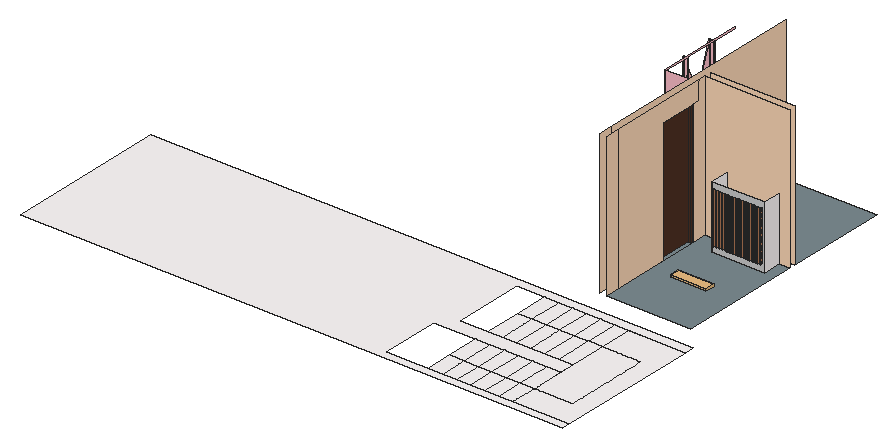
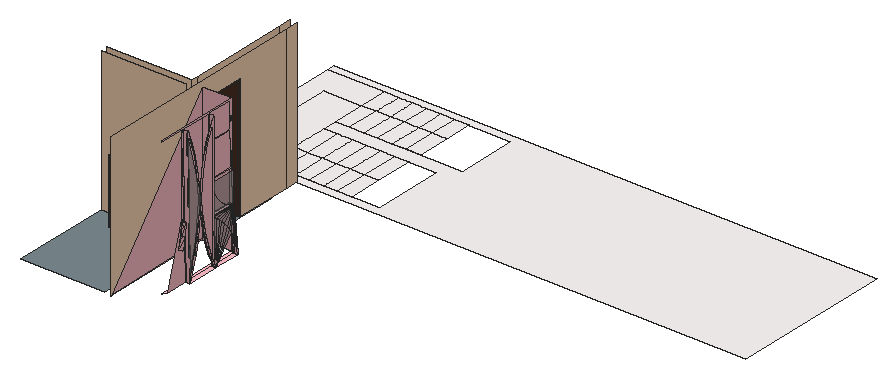
# SketchUp Ruby script. Lengths in inches.
U = 1.inch
M = Sketchup.active_model
def pt(a) = Geom::Point3d.new(a.map { |v| v * U })
def face(e, loops, mat)
  f = e.add_face(loops[0].map { |a| pt(a) })
  loops[1..].each { |l| e.add_face(l.map { |a| pt(a) }).erase! }
  f.material = f.back_material = mat if mat
  f
end
# faces: each face lists its corners as indices into pts; further lists are holes
def faces(e, pts, list, mat = nil) = list.each { |f| face(e, (f[0].is_a?(Array) ? f : [f]).map { |l| l.map { |i| pts[i] } }, mat) }
# xy, xz, yz: faces in a plane at the given z, y or x. An outline is a flat list of corners, or four numbers for a rectangle; further outlines are holes
def ring(l) = l.size == 4 ? [[l[0], l[1]], [l[2], l[1]], [l[2], l[3]], [l[0], l[3]]] : l.each_slice(2).to_a
def flat(e, list, mat, &to3) = list.each { |f| face(e, (f[0].is_a?(Array) ? f : [f]).map { |l| ring(l).map { |u, v| to3.(u, v) } }, mat) }
def xy(e, z, list, mat = nil) = flat(e, list, mat) { |x, y| [x, y, z] }
def xz(e, y, list, mat = nil) = flat(e, list, mat) { |x, z| [x, y, z] }
def yz(e, x, list, mat = nil) = flat(e, list, mat) { |y, z| [x, y, z] }
def lines(e, pts, list) = list.each { |a, b| e.add_line(pt(pts[a]), pt(pts[b])) }
# prism: a flat outline (further loops are holes) pulled along v
def prism(e, loops, v, mat = nil)
  f = face(e, loops, mat); d = Geom::Vector3d.new(v.map { |x| x * U })
  f.pushpull(f.normal.samedirection?(d) ? d.length : -d.length)
end
def box(e, o, s, mat = nil) = prism(e, [[o, [o[0] + s[0], o[1], o[2]], [o[0] + s[0], o[1] + s[1], o[2]], [o[0], o[1] + s[1], o[2]]]], [0, 0, s[2]], mat)
def at(x, y, z, deg = 0) = Geom::Transformation.translation(pt([x, y, z])) * Geom::Transformation.rotation(ORIGIN, Z_AXIS, deg.degrees)
def axes(o, x, y, z) = Geom::Transformation.new([*x, 0, *y, 0, *z, 0, *pt(o).to_a, 1])
def part(name) = M.definitions.add(name)
# library, detail: a bought-in or finely detailed component or shape, given as its bounding box
def library(name, o, s) = part(name).tap { |d| box(d.entities, o, s) }
def detail(e, o, s) = box(e.add_group.entities, o, s)
def put(e, d, t, mat = nil) = e.add_instance(d, t).tap { |i| i.material = mat if mat }
def group(e, t, mat = nil) = e.add_group.tap { |g| g.transformation = t; g.material = mat if mat }.entities
root = M.entities
M.materials.add("Polis06_194").color = [79, 50, 36]
M.materials.add("[0006_Pink]").color = [255, 192, 203]
M.materials.add("[0007_MistyRose]").color = [255, 228, 225]
M.materials.add("[0010_Snow]").color = [255, 250, 250]
M.materials.add("[0027_PeachPuff]").color = [255, 218, 185]
M.materials.add("[Carrera Marble]").color = [207, 207, 207]
M.materials.add("[Concrete Pavers Block Multi]").color = [124, 140, 145]
M.materials.add("[Translucent Glass Gray]").color = [128, 128, 128]
M.materials["[Translucent Glass Gray]"].alpha = 0.5
M.materials.add("[Wood Veneer 02]").color = [190, 128, 91]
c1 = part("Interior door")
xy(c1.entities,0,[[0,0,4.72,1.18],[0,34.25,4.72,35.43]],"Polis06_194")
xy(c1.entities,85.26,[[0,1.18,4.72,34.25]],"Polis06_194")
xy(c1.entities,86.61,[[0,0,4.72,35.43]],"Polis06_194")
xz(c1.entities,0,[[0,0,4.72,86.61]],"Polis06_194")
xz(c1.entities,1.18,[[0,0,2.36,85.26],[2.36,0,4.72,85.26]],"Polis06_194")
xz(c1.entities,34.25,[[0,0,4.72,85.26]],"Polis06_194")
xz(c1.entities,35.43,[[0,0,4.72,86.61]],"Polis06_194")
yz(c1.entities,0,[[0,0,1.18,86.61],[34.25,0,35.43,86.61],[1.18,85.26,34.25,86.61]],"Polis06_194")
yz(c1.entities,2.36,[[1.18,0,34.25,0,34.25,85.21,1.18,85.26]],"Polis06_194")
yz(c1.entities,4.72,[[0,0,1.18,86.61],[34.25,0,35.43,86.61],[1.18,85.26,34.25,86.61]],"Polis06_194")
c2 = library("toilet 2",[0.13,0,0],[30.44,8.22,2])
xy(root,-7.5625,[[109.5625,0,571.5625,0,571.5625,6.25,415.5625,6.25,415.5625,57.9375,523.5625,57.9375,523.5625,70.375,427.5625,70.375,427.5625,130.875,571.5625,130.875,571.5625,138.9375,109.5625,138.9375],[451.5625,6.25,463.5625,29.875],[463.5625,6.25,475.5625,29.875],[475.5625,6.25,487.5625,29.875],[487.5625,6.25,499.5625,29.875],
  [499.5625,6.25,511.5625,29.875],[511.5625,6.25,523.5625,29.875],[523.5625,6.25,571.5625,6.25,571.5625,130.875,523.5625,130.875,523.5625,102.3125,556.33,102.3125,556.33,29.875,523.5625,29.875],[451.5625,29.875,463.5625,57.9375],[463.5625,29.875,475.5625,57.9375],
  [475.5625,29.875,487.5625,57.9375],[487.5625,29.875,499.5625,57.9375],[499.5625,29.875,511.5625,57.9375],[511.5625,29.875,523.5625,57.9375],[523.5625,29.875,556.33,102.3125],
  [451.5625,70.375,463.5625,102.3125],[463.5625,70.375,475.5625,102.3125],[475.5625,70.375,487.5625,102.3125],[487.5625,70.375,499.5625,102.3125],[499.5625,70.375,511.5625,102.3125],
  [511.5625,70.375,523.5625,102.3125],[451.5625,102.3125,463.5625,130.875],[463.5625,102.3125,475.5625,130.875],[475.5625,102.3125,487.5625,130.875],[487.5625,102.3125,499.5625,130.875],
  [499.5625,102.3125,511.5625,130.875],[511.5625,102.3125,523.5625,130.875]],"[0010_Snow]")
xy(root,0,[[508.61,237.66,553.2,252.9375],[500.21,258.9375,543.78,274.78]],"[0010_Snow]")
xy(root,0,[[484.5625,240.51,490.5625,246.2]],"[0027_PeachPuff]")
xy(root,0,[[490.5625,147.9375,562.5625,147.9375,562.5625,252.9375,553.2,252.9375,553.2,237.66,508.61,237.66,508.61,252.9375,490.5625,252.9375],[483.52,177.19,490.5625,240.51],[490.5625,258.9375,500.21,258.9375,500.21,274.78,543.78,274.78,543.78,258.9375,562.5625,258.9375,562.5625,345.21,490.5625,345.21]],"[Concrete Pavers Block Multi]")
xy(root,0.5,[[453.17,250.71,456.54,272.96],[453.17,273.46,456.54,301.21]],"[0006_Pink]")
xy(root,5.99,[[510.4375,236.375,511.58,237.09],[512.87,236.375,514.01,237.09],[515.3,236.375,516.4375,237.09],[517.73,236.375,518.87,237.09],[520.16,236.375,521.3,237.09],
  [522.59,236.375,523.73,237.09],[525.02,236.375,526.16,237.09],[527.45,236.375,528.59,237.09],[529.88,236.375,531.02,237.09],[531.83,236.375,532.97,237.09],
  [534.125,236.375,535.26,237.09],[536.42,236.375,537.55,237.09],[538.71,236.375,539.85,237.09],[541,236.375,542.14,237.09],[543.3,236.375,544.43,237.09],
  [545.59,236.375,546.73,237.09],[547.88,236.375,549.02,237.09],[550.18,236.375,551.3125,237.09],[510.4375,237.09,531.02,237.66],[531.51,237.09,551.3125,237.66]],"[0010_Snow]")
xy(root,6.2,[[502.06,274.78,521.41,275.36],[521.88,274.78,542,275.36],[502.06,275.36,503.17,276.11],[504.3,275.36,505.41,276.11],[506.54,275.36,507.65,276.11],
  [508.78,275.36,509.89,276.11],[511.02,275.36,512.13,276.11],[513.26,275.36,514.37,276.11],[515.5,275.36,516.61,276.11],[517.74,275.36,518.85,276.11],
  [519.98,275.36,521.09,276.11],[521.88,275.36,522.99,276.11],[524.26,275.36,525.37,276.11],[526.63,275.36,527.74,276.11],[529.01,275.36,530.12,276.11],
  [531.38,275.36,532.5,276.11],[533.76,275.36,534.87,276.11],[536.13,275.36,537.25,276.11],[538.51,275.36,539.62,276.11],[540.89,275.36,542,276.11]],"[0010_Snow]")
xy(root,37.375,[[456.0625,250.71,459.4375,272.96]],"[0006_Pink]")
xy(root,37.875,[[456.0625,250.71,459.4375,272.96]],"[0006_Pink]")
xz(root,207.77,[[484.5625,0,490.5625,105.5625]],"[0027_PeachPuff]")
xz(root,236.375,[[510.4375,5.99,511.58,48.56],[512.87,5.99,514.01,48.56],[515.3,5.99,516.4375,48.56],[517.73,5.99,518.87,48.56],[520.16,5.99,521.3,48.56],
  [522.59,5.99,523.73,48.56],[525.02,5.99,526.16,48.56],[527.45,5.99,528.59,48.56],[529.88,5.99,531.02,48.56],[531.83,5.99,532.97,48.56],
  [534.125,5.99,535.26,48.56],[536.42,5.99,537.55,48.56],[538.71,5.99,539.85,48.56],[541,5.99,542.14,48.56],[543.3,5.99,544.43,48.56],
  [545.59,5.99,546.73,48.56],[547.88,5.99,549.02,48.56],[550.18,5.99,551.3125,48.56]],"[Wood Veneer 02]")
xz(root,237.09,[[510.4375,5.99,511.58,48.56],[511.58,5.99,512.87,48.56],[512.87,5.99,514.01,48.56],[514.01,5.99,515.3,48.56],[515.3,5.99,516.4375,48.56],
  [516.4375,5.99,517.73,48.56],[517.73,5.99,518.87,48.56],[518.87,5.99,520.16,48.56],[520.16,5.99,521.3,48.56],[521.3,5.99,522.59,48.56],
  [522.59,5.99,523.73,48.56],[523.73,5.99,525.02,48.56],[525.02,5.99,526.16,48.56],[526.16,5.99,527.45,48.56],[527.45,5.99,528.59,48.56],
  [529.88,5.99,531.02,48.56],[531.51,5.99,531.83,48.56],[531.83,5.99,532.97,48.56],[532.97,5.99,534.125,48.56],[534.125,5.99,535.26,48.56],
  [535.26,5.99,536.42,48.56],[536.42,5.99,537.55,48.56],[537.55,5.99,538.71,48.56],[538.71,5.99,539.85,48.56],[539.85,5.99,541,48.56],
  [541,5.99,542.14,48.56],[542.14,5.99,543.3,48.56],[543.3,5.99,544.43,48.56],[544.43,5.99,545.59,48.56],[545.59,5.99,546.73,48.56],
  [546.73,5.99,547.88,48.56],[547.88,5.99,549.02,48.56],[549.02,5.99,550.18,48.56],[550.18,5.99,551.3125,48.56]],"[0010_Snow]")
xz(root,237.09,[[528.59,5.99,529.88,48.56]],"[Wood Veneer 02]")
xz(root,237.66,[[[508.61,0,553.2,53.66],[510.4375,5.99,531.02,48.56],[531.51,5.99,551.3125,48.56]]],"[Carrera Marble]")
xz(root,240.51,[[484.5625,0,490.5625,105.5625]],"[0027_PeachPuff]")
xz(root,249.21,[[459.4375,0,484.5625,0,484.33,0.5,484.5625,116.8125,459.4375,116.8125]],"[0006_Pink]")
xz(root,250.71,[[453.17,0.5,456.54,0.5,457.47,37.375,456.0625,37.375],[456.54,0.5,459.4375,37.375,457.47,37.375],[457.47,37.375,459.4375,37.375,459.4375,37.875,457.48,37.875],[456.0625,37.875,457.48,37.875,458.13,63.875,456.0625,63.875],[457.48,37.875,459.4375,37.875,459.4375,63.875,458.13,63.875]],"[0006_Pink]")
xz(root,252.9375,[[490.5625,0,562.5625,121.1875]],"[0027_PeachPuff]")
xz(root,252.9375,[[508.61,0,553.2,53.66]],"[Wood Veneer 02]")
xz(root,258.9375,[[490.5625,0,562.5625,121.1875]],"[0027_PeachPuff]")
xz(root,258.9375,[[500.21,0,543.78,55.54]],"[Wood Veneer 02]")
xz(root,272.96,[[453.17,0.5,456.0625,37.375,459.4375,37.375,456.54,0.5],[456.0625,37.875,459.4375,63.875]],"[0006_Pink]")
xz(root,273.46,[[455.3125,0.5,456.54,0.5,459.4375,115.8125,456.0625,115.8125,456.0625,114.75,455.3125,114.75]],"[0006_Pink]")
xz(root,273.86,[[455.3125,2.32,456.0625,112.97]],"[0006_Pink]")
xz(root,274.78,[[[500.21,0,543.78,55.54],[521.88,6.2,542,50.26],[502.06,6.2,521.41,50.26]]],"[0010_Snow]")
xz(root,275.36,[[502.06,6.2,503.17,50.26],[503.17,6.2,504.3,50.26],[504.3,6.2,505.41,50.26],[505.41,6.2,506.54,50.26],[506.54,6.2,507.65,50.26],
  [507.65,6.2,508.78,50.26],[508.78,6.2,509.89,50.26],[509.89,6.2,511.02,50.26],[511.02,6.2,512.13,50.26],[512.13,6.2,513.26,50.26],
  [513.26,6.2,514.37,50.26],[514.37,6.2,515.5,50.26],[515.5,6.2,516.61,50.26],[516.61,6.2,517.74,50.26],[517.74,6.2,518.85,50.26],
  [518.85,6.2,519.98,50.26],[519.98,6.2,521.09,50.26],[521.09,6.2,521.41,50.26],[521.88,6.2,522.99,50.26],[522.99,6.2,524.26,50.26],
  [524.26,6.2,525.37,50.26],[525.37,6.2,526.63,50.26],[526.63,6.2,527.74,50.26],[527.74,6.2,529.01,50.26],[529.01,6.2,530.12,50.26],
  [530.12,6.2,531.38,50.26],[531.38,6.2,532.5,50.26],[532.5,6.2,533.76,50.26],[533.76,6.2,534.87,50.26],[534.87,6.2,536.13,50.26],
  [536.13,6.2,537.25,50.26],[537.25,6.2,538.51,50.26],[538.51,6.2,539.62,50.26],[539.62,6.2,540.89,50.26]],"[0010_Snow]")
xz(root,275.36,[[540.89,6.2,542,50.26]],"[Wood Veneer 02]")
xz(root,276.11,[[502.06,6.2,503.17,50.26],[504.3,6.2,505.41,50.26],[506.54,6.2,507.65,50.26],[508.78,6.2,509.89,50.26],[511.02,6.2,512.13,50.26],
  [513.26,6.2,514.37,50.26],[515.5,6.2,516.61,50.26],[517.74,6.2,518.85,50.26],[519.98,6.2,521.09,50.26],[521.88,6.2,522.99,50.26],
  [524.26,6.2,525.37,50.26],[526.63,6.2,527.74,50.26],[529.01,6.2,530.12,50.26],[531.38,6.2,532.5,50.26],[533.76,6.2,534.87,50.26],
  [536.13,6.2,537.25,50.26],[538.51,6.2,539.62,50.26],[540.89,6.2,542,50.26]],"[Wood Veneer 02]")
xz(root,300.68,[[455.37,3.27,456.06,113.05]],"[0006_Pink]")
xz(root,301.21,[[453.17,0.5,455.375,0.5,455.375,115.8125],[453.17,0.5,455.375,115.8125,456.0625,115.8125],[453.17,0.5,456.0625,115.8125,459.4375,115.8125,456.54,0.5]],"[0006_Pink]")
xz(root,301.65,[[453.1,0.5,456.54,0.5,459.4375,115.8125,456,115.8125]],"[0006_Pink]")
xz(root,301.71,[[456.54,0.5,459.4375,115.8125,459.4375,46.85]],"[0006_Pink]")
yz(root,455.3125,[[[273.46,0.5,273.46,114.75,277.22,106.79,280.75,97.45,283.53,87.87,285.54,78.09,286.77,68.1875,287.21,58.22,286.86,48.24,285.71,38.33,283.79,28.54,281.09,18.93,277.64,9.5625],[273.86,2.32,277.27,9.71,280.71,19.05,283.4,28.63,285.32,38.39,286.46,48.27,286.81,58.22,286.37,68.15,285.15,78.03,283.14,87.77,280.37,97.33,276.85,106.63,273.86,112.97]]],"[0006_Pink]")
yz(root,456.0625,[[273.86,2.32,273.86,112.97,276.85,106.63,280.37,97.33,283.14,87.77,285.15,78.03,286.37,68.15,286.81,58.22,286.46,48.27,285.32,38.39,283.4,28.63,280.71,19.05,277.27,9.71]],"[0006_Pink]")
yz(root,456.0625,[[250.71,37.875,250.71,63.875,272.96,63.875,272.63,60.83,271.97,57.83,270.99,54.93,269.7,52.15,268.11,49.53,266.25,47.1,264.13,44.88,261.79,42.91,259.24,41.2,256.53,39.78,253.67,38.67],[250.71,37.875,253.67,38.67,256.53,39.78,259.24,41.2,261.79,42.91,264.13,44.88,266.25,47.1,268.11,49.53,269.7,52.15,270.99,54.93,271.97,57.83,272.63,60.83,272.96,63.875,272.96,37.875]],"[Translucent Glass Gray]")
yz(root,459.4375,[[249.21,0,249.21,116.8125,323.46,116.8125,323.46,115.8125,273.46,115.8125,272.96,37.375,250.71,37.375,250.71,37.875,272.96,37.875,272.96,63.875,250.71,63.875,250.71,64.375,272.96,64.375,272.96,93.125,250.71,93.125,250.71,93.625,272.96,93.625,272.96,115.8125,250.71,115.8125]],"[0006_Pink]")
yz(root,484.5625,[[147.9375,0,159.9375,121.1875],[159.9375,0,159.9375,121.1875,345.9375,121.1875,345.9375,0,240.51,0,240.51,105.5625,207.77,105.5625,207.77,0]],"[0027_PeachPuff]")
yz(root,490.5625,[[147.9375,0,159.9375,121.1875],[159.9375,0,207.77,0,207.77,105.5625,246.2,105.5625,246.2,121.1875,159.9375,121.1875],[240.51,0,252.9375,0,252.9375,121.1875,246.2,121.1875,246.2,105.5625,240.51,105.5625]],"[0027_PeachPuff]")
yz(root,500.21,[[258.9375,0,274.78,55.54]],"[0010_Snow]")
yz(root,502.06,[[274.78,6.2,275.36,50.26]],"[0010_Snow]")
yz(root,502.06,[[275.36,6.2,276.11,50.26]],"[Wood Veneer 02]")
yz(root,503.17,[[275.36,6.2,276.11,50.26]],"[Wood Veneer 02]")
yz(root,504.3,[[275.36,6.2,276.11,50.26]],"[Wood Veneer 02]")
yz(root,505.41,[[275.36,6.2,276.11,50.26]],"[Wood Veneer 02]")
yz(root,506.54,[[275.36,6.2,276.11,50.26]],"[Wood Veneer 02]")
yz(root,507.65,[[275.36,6.2,276.11,50.26]],"[Wood Veneer 02]")
yz(root,508.61,[[237.66,0,252.9375,53.66]],"[0010_Snow]")
yz(root,508.78,[[275.36,6.2,276.11,50.26]],"[Wood Veneer 02]")
yz(root,509.89,[[275.36,6.2,276.11,50.26]],"[Wood Veneer 02]")
yz(root,510.4375,[[237.09,5.99,237.66,48.56]],"[0010_Snow]")
yz(root,510.4375,[[236.375,5.99,237.09,48.56]],"[Wood Veneer 02]")
yz(root,511.02,[[275.36,6.2,276.11,50.26]],"[Wood Veneer 02]")
yz(root,511.58,[[236.375,5.99,237.09,48.56]],"[Wood Veneer 02]")
yz(root,512.13,[[275.36,6.2,276.11,50.26]],"[Wood Veneer 02]")
yz(root,512.87,[[236.375,5.99,237.09,48.56]],"[Wood Veneer 02]")
yz(root,513.26,[[275.36,6.2,276.11,50.26]],"[Wood Veneer 02]")
yz(root,514.01,[[236.375,5.99,237.09,48.56]],"[Wood Veneer 02]")
yz(root,514.37,[[275.36,6.2,276.11,50.26]],"[Wood Veneer 02]")
yz(root,515.3,[[236.375,5.99,237.09,48.56]],"[Wood Veneer 02]")
yz(root,515.5,[[275.36,6.2,276.11,50.26]],"[Wood Veneer 02]")
yz(root,516.4375,[[236.375,5.99,237.09,48.56]],"[Wood Veneer 02]")
yz(root,516.61,[[275.36,6.2,276.11,50.26]],"[Wood Veneer 02]")
yz(root,517.73,[[236.375,5.99,237.09,48.56]],"[Wood Veneer 02]")
yz(root,517.74,[[275.36,6.2,276.11,50.26]],"[Wood Veneer 02]")
yz(root,518.85,[[275.36,6.2,276.11,50.26]],"[0010_Snow]")
yz(root,518.87,[[236.375,5.99,237.09,48.56]],"[Wood Veneer 02]")
yz(root,519.98,[[275.36,6.2,276.11,50.26]],"[Wood Veneer 02]")
yz(root,520.16,[[236.375,5.99,237.09,48.56]],"[Wood Veneer 02]")
yz(root,521.09,[[275.36,6.2,276.11,50.26]],"[Wood Veneer 02]")
yz(root,521.3,[[236.375,5.99,237.09,48.56]],"[Wood Veneer 02]")
yz(root,521.41,[[274.78,6.2,275.36,50.26]],"[0010_Snow]")
yz(root,521.88,[[274.78,6.2,275.36,50.26]],"[0010_Snow]")
yz(root,521.88,[[275.36,6.2,276.11,50.26]],"[Wood Veneer 02]")
yz(root,522.59,[[236.375,5.99,237.09,48.56]],"[Wood Veneer 02]")
yz(root,522.99,[[275.36,6.2,276.11,50.26]],"[Wood Veneer 02]")
yz(root,523.73,[[236.375,5.99,237.09,48.56]],"[Wood Veneer 02]")
yz(root,524.26,[[275.36,6.2,276.11,50.26]],"[Wood Veneer 02]")
yz(root,525.02,[[236.375,5.99,237.09,48.56]],"[Wood Veneer 02]")
yz(root,525.37,[[275.36,6.2,276.11,50.26]],"[Wood Veneer 02]")
yz(root,526.16,[[236.375,5.99,237.09,48.56]],"[Wood Veneer 02]")
yz(root,526.63,[[275.36,6.2,276.11,50.26]],"[Wood Veneer 02]")
yz(root,527.45,[[236.375,5.99,237.09,48.56]],"[Wood Veneer 02]")
yz(root,527.74,[[275.36,6.2,276.11,50.26]],"[Wood Veneer 02]")
yz(root,528.59,[[236.375,5.99,237.09,48.56]],"[Wood Veneer 02]")
yz(root,529.01,[[275.36,6.2,276.11,50.26]],"[Wood Veneer 02]")
yz(root,529.88,[[236.375,5.99,237.09,48.56]],"[Wood Veneer 02]")
yz(root,530.12,[[275.36,6.2,276.11,50.26]],"[Wood Veneer 02]")
yz(root,531.02,[[237.09,5.99,237.66,48.56]],"[0010_Snow]")
yz(root,531.02,[[236.375,5.99,237.09,48.56]],"[Wood Veneer 02]")
yz(root,531.38,[[275.36,6.2,276.11,50.26]],"[Wood Veneer 02]")
yz(root,531.51,[[237.09,5.99,237.66,48.56]],"[0010_Snow]")
yz(root,531.83,[[236.375,5.99,237.09,48.56]],"[Wood Veneer 02]")
yz(root,532.5,[[275.36,6.2,276.11,50.26]],"[Wood Veneer 02]")
yz(root,532.97,[[236.375,5.99,237.09,48.56]],"[Wood Veneer 02]")
yz(root,533.76,[[275.36,6.2,276.11,50.26]],"[Wood Veneer 02]")
yz(root,534.125,[[236.375,5.99,237.09,48.56]],"[Wood Veneer 02]")
yz(root,534.87,[[275.36,6.2,276.11,50.26]],"[Wood Veneer 02]")
yz(root,535.26,[[236.375,5.99,237.09,48.56]],"[Wood Veneer 02]")
yz(root,536.13,[[275.36,6.2,276.11,50.26]],"[Wood Veneer 02]")
yz(root,536.42,[[236.375,5.99,237.09,48.56]],"[Wood Veneer 02]")
yz(root,537.25,[[275.36,6.2,276.11,50.26]],"[Wood Veneer 02]")
yz(root,537.55,[[236.375,5.99,237.09,48.56]],"[Wood Veneer 02]")
yz(root,538.51,[[275.36,6.2,276.11,50.26]],"[Wood Veneer 02]")
yz(root,538.71,[[236.375,5.99,237.09,48.56]],"[Wood Veneer 02]")
yz(root,539.62,[[275.36,6.2,276.11,50.26]],"[Wood Veneer 02]")
yz(root,539.85,[[236.375,5.99,237.09,48.56]],"[Wood Veneer 02]")
yz(root,540.89,[[275.36,6.2,276.11,50.26]],"[Wood Veneer 02]")
yz(root,541,[[236.375,5.99,237.09,48.56]],"[Wood Veneer 02]")
yz(root,542,[[274.78,6.2,275.36,50.26]],"[0010_Snow]")
yz(root,542,[[275.36,6.2,276.11,50.26]],"[Wood Veneer 02]")
yz(root,542.14,[[236.375,5.99,237.09,48.56]],"[Wood Veneer 02]")
yz(root,543.3,[[236.375,5.99,237.09,48.56]],"[Wood Veneer 02]")
yz(root,543.78,[[258.9375,0,274.78,55.54]],"[0010_Snow]")
yz(root,544.43,[[236.375,5.99,237.09,48.56]],"[Wood Veneer 02]")
yz(root,545.59,[[236.375,5.99,237.09,48.56]],"[Wood Veneer 02]")
yz(root,546.73,[[236.375,5.99,237.09,48.56]],"[Wood Veneer 02]")
yz(root,547.88,[[236.375,5.99,237.09,48.56]],"[Wood Veneer 02]")
yz(root,549.02,[[236.375,5.99,237.09,48.56]],"[Wood Veneer 02]")
yz(root,550.18,[[236.375,5.99,237.09,48.56]],"[Wood Veneer 02]")
yz(root,551.3125,[[237.09,5.99,237.66,48.56]],"[0010_Snow]")
yz(root,551.3125,[[236.375,5.99,237.09,48.56]],"[Wood Veneer 02]")
yz(root,553.2,[[237.66,0,252.9375,53.66]],"[0010_Snow]")
p = [[456.54,301.65,0.5],[456.54,301.71,0.5],[456.54,320.52,0.5],[459.4375,323.46,0],[459.4375,249.21,0],[456.54,250.71,0.5],
  [456.54,272.96,0.5],[456.54,273.46,0.5],[456.54,301.21,0.5],[459.4375,250.71,115.8125],[458.88,250.71,93.625],[458.87,250.71,93.125],
  [458.15,250.71,64.375],[458.13,250.71,63.875],[457.48,250.71,37.875],[457.47,250.71,37.375],[484.5625,249.21,0],[484.5625,345.9375,0],
  [484.33,249.21,0.5],[484.5625,249.21,116.8125],[453.17,250.71,0.5],[456.0625,250.71,37.375],[453.39,251.08,4.22],[454.61,257.28,21.6875],
  [453.17,272.96,0.5],[454.36,255.48,18.42],[454.87,259.33,24.8],[455.11,261.63,27.74],[455.36,264.16,30.49],[455.6,266.91,33.02],
  [455.84,269.84,35.32],[456.0625,272.96,37.375],[459.4375,273.46,115.8125],[459.4375,272.96,37.375],[455.3125,273.46,0.5],[455.3125,277.64,9.5625],
  [453.4,277.64,9.5625],[453.17,273.46,0.5],[456.0625,301.21,115.8125],[453.17,301.21,0.5],[454.63,287.21,58.22],[455.36,297.53,106.63],
  [455.375,301.21,115.8125],[455.375,301.21,0.5],[455.36,297.53,9.68],[455.34,294.5,19.09],[455.33,292.12,28.69],[455.32,290.42,38.44],
  [455.3125,289.39,48.27],[455.3125,289.05,58.16],[455.3125,289.39,68.04],[455.32,290.42,77.88],[455.33,292.12,87.62],[455.34,294.5,97.22],
  [455.33,292.65,28.8],[455.34,295.01,19.24],[455.36,298.04,9.86],[455.37,300.68,3.27],[455.37,300.68,113.05],[455.36,298.04,106.45],
  [455.34,295.01,97.07],[455.33,292.65,87.51],[455.32,290.95,77.8],[455.32,289.92,68],[455.32,289.58,58.16],[455.32,289.92,48.31],
  [455.32,290.95,38.51],[453.38,297.53,9.68],[456.05,298.03,9.86],[456.06,300.68,3.27],[459.4375,301.21,115.8125],[459.4375,301.65,115.8125],
  [459.4375,301.71,115.8125],[459.4375,301.71,46.85],[456.0625,273.86,2.32],[456.0625,277.27,9.71],[455.3125,277.27,9.71],[455.3125,273.86,2.32],
  [456.03,295.01,19.24],[456.02,292.64,28.8],[456.01,290.94,38.51],[456,289.92,48.31],[456,289.58,58.16],[456,289.92,68],
  [456.01,290.94,77.8],[456.02,292.64,87.51],[456.03,295.01,97.07],[456.05,298.03,106.45],[456.06,300.68,113.05],[453.63,251.74,7.89],
  [453.87,252.7,11.5],[455.3125,281.09,18.93],[453.63,281.09,18.93],[456.0625,280.71,19.05],[455.3125,280.71,19.05],[453.6,294.49,19.09],
  [454.11,253.95,15.01],[455.3125,283.79,28.54],[453.88,283.79,28.54],[456.0625,283.4,28.63],[455.3125,283.4,28.63],[453.83,292.12,28.69],
  [453.8,308.31,28.26],[454.05,306.07,38.09],[456,309.18,28.5],[455.3125,285.71,38.33],[454.125,285.72,38.33],[456,306.96,38.25],
  [456.75,306.96,38.25],[456.75,309.18,28.5],[456.0625,285.32,38.39],[455.3125,285.32,38.39],[454.0625,290.41,38.4375],[454.3,304.72,48.08],
  [456,305.625,48.16],[456.75,305.625,48.16],[454.375,286.86,48.24],[455.3125,286.86,48.24],[456.0625,286.46,48.27],[455.3125,286.46,48.27],
  [454.31,289.38,48.27]]
faces(root,p,[[0,1,2,3,4,5,6,7,8],[16,17,18],[19,18,17],[32,7,6],[6,33,32],[34,35,36,37],[[41,42,43,44,45,46,47,48,49,50,51,52,53],[54,55,56,57,58,59,60,61,62,63,64,65,66]],[67,39,68],
  [39,67,44,43],[69,68,39],[39,38,69],[70,71,0,8],[0,1,72,71],[1,2,73],[74,75,76,77],[78,79,80,81,82,83,84,85,86,87,88,69,68],
  [68,69,57,56],[88,69,38],[35,91,92,36],[75,93,94,76],[95,67,78],[67,95,45,44],[68,78,67],[78,68,56,55],
  [91,97,98,92],[93,99,100,94],[101,95,79],[95,101,46,45],[78,79,95],[79,78,55,54],[102,103,104],[97,105,106,98],
  [107,104,103],[108,107,104,109],[99,110,111,100],[101,112,46],[112,101,80],[47,46,112],[79,80,101],[80,79,54,66],
  [103,113,107],[114,107,113],[115,114,107,108],[116,106,117],[105,117,106],[110,118,119,111],[112,120,47],[120,112,81],
  [48,47,120],[80,81,112],[81,80,66,65]],"[0006_Pink]")
faces(root,p,[[9,10,11,12,13,14,15,5,4]],"[0007_MistyRose]")
faces(root,p,[[20,21,22],[23,24,25],[26,24,23],[27,24,26],[28,24,27],[29,24,28],[30,24,29],[31,24,30],
  [38,39,40],[89,22,21],[90,89,21],[96,90,21],[25,96,21],[23,25,21],[26,23,21],[27,26,21],
  [28,27,21],[29,28,21],[30,29,21],[31,30,21]],"[Translucent Glass Gray]")
put(root,c1,axes([484.8,207.77,0],[0.95,0,0],[0,0.912,0],[0,0,1.21877]),"[0006_Pink]")
put(root,c2,at(508.21,193.79,0))
